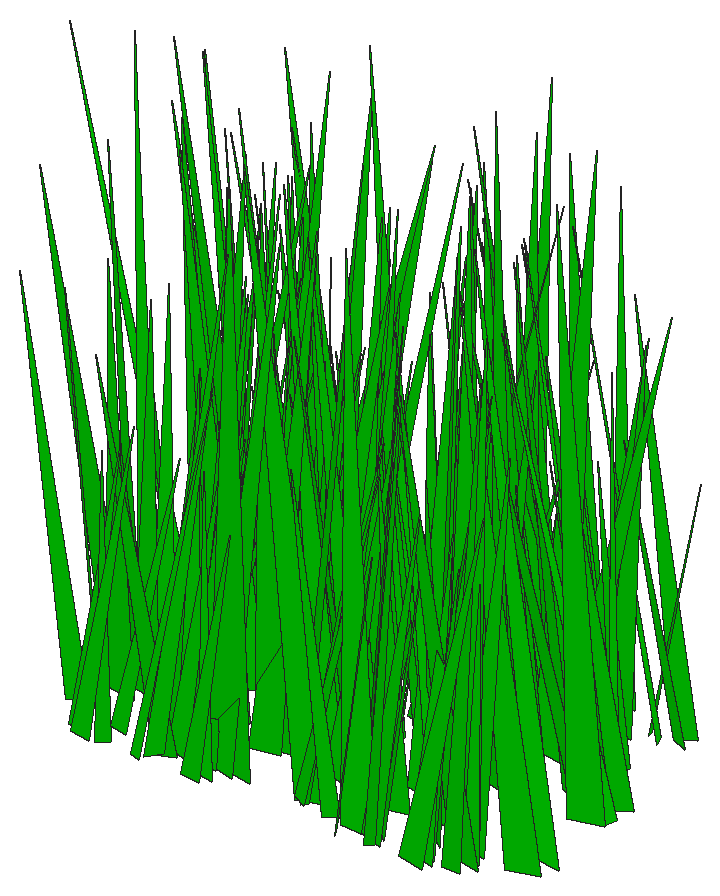
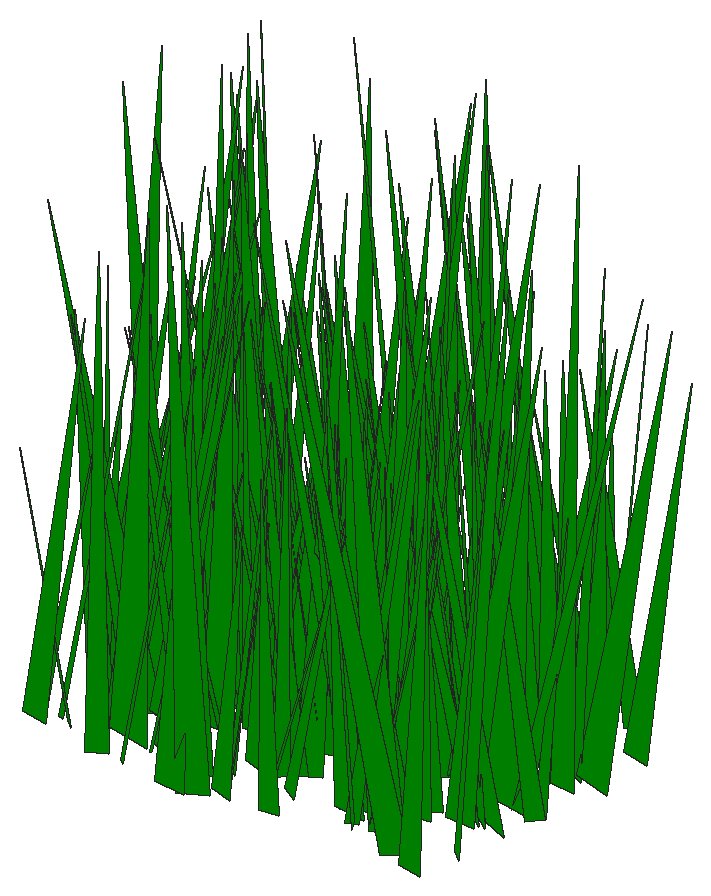
# SketchUp Ruby script. Lengths in inches.
U = 1.inch
M = Sketchup.active_model
def pt(a) = Geom::Point3d.new(a.map { |v| v * U })
def face(e, loops, mat)
  f = e.add_face(loops[0].map { |a| pt(a) })
  loops[1..].each { |l| e.add_face(l.map { |a| pt(a) }).erase! }
  f.material = f.back_material = mat if mat
  f
end
# faces: each face lists its corners as indices into pts; further lists are holes
def faces(e, pts, list, mat = nil) = list.each { |f| face(e, (f[0].is_a?(Array) ? f : [f]).map { |l| l.map { |i| pts[i] } }, mat) }
# xy, xz, yz: faces in a plane at the given z, y or x. An outline is a flat list of corners, or four numbers for a rectangle; further outlines are holes
def ring(l) = l.size == 4 ? [[l[0], l[1]], [l[2], l[1]], [l[2], l[3]], [l[0], l[3]]] : l.each_slice(2).to_a
def flat(e, list, mat, &to3) = list.each { |f| face(e, (f[0].is_a?(Array) ? f : [f]).map { |l| ring(l).map { |u, v| to3.(u, v) } }, mat) }
def xy(e, z, list, mat = nil) = flat(e, list, mat) { |x, y| [x, y, z] }
def xz(e, y, list, mat = nil) = flat(e, list, mat) { |x, z| [x, y, z] }
def yz(e, x, list, mat = nil) = flat(e, list, mat) { |y, z| [x, y, z] }
def lines(e, pts, list) = list.each { |a, b| e.add_line(pt(pts[a]), pt(pts[b])) }
# prism: a flat outline (further loops are holes) pulled along v
def prism(e, loops, v, mat = nil)
  f = face(e, loops, mat); d = Geom::Vector3d.new(v.map { |x| x * U })
  f.pushpull(f.normal.samedirection?(d) ? d.length : -d.length)
end
def box(e, o, s, mat = nil) = prism(e, [[o, [o[0] + s[0], o[1], o[2]], [o[0] + s[0], o[1] + s[1], o[2]], [o[0], o[1] + s[1], o[2]]]], [0, 0, s[2]], mat)
def at(x, y, z, deg = 0) = Geom::Transformation.translation(pt([x, y, z])) * Geom::Transformation.rotation(ORIGIN, Z_AXIS, deg.degrees)
def axes(o, x, y, z) = Geom::Transformation.new([*x, 0, *y, 0, *z, 0, *pt(o).to_a, 1])
def part(name) = M.definitions.add(name)
# library, detail: a bought-in or finely detailed component or shape, given as its bounding box
def library(name, o, s) = part(name).tap { |d| box(d.entities, o, s) }
def detail(e, o, s) = box(e.add_group.entities, o, s)
def put(e, d, t, mat = nil) = e.add_instance(d, t).tap { |i| i.material = mat if mat }
def group(e, t, mat = nil) = e.add_group.tap { |g| g.transformation = t; g.material = mat if mat }.entities
root = M.entities
M.materials.add("[Color G06]").color = [0, 204, 0]
c1 = part("fur_instance\#9")
p = [[0.8125,0,1.79],[0.67,-0.02,1.48],[0,-0.11,0],[0,0.11,0]]
faces(c1.entities,p,[[0,1,2,3]])
put(root,c1,axes([12.96,21.07,4.28],[-5.73012,0.26102,0.16531],[1.85665,0.79674,-0.75835],[0.26235,0.0625,8.97748]),"[Color G06]")
put(root,c1,axes([12.26,19.0625,4.28],[-1.91963,-0.63161,0.80341],[-4.54214,0.25727,-1.00806],[-0.41693,0.10528,7.28303]),"[Color G06]")
put(root,c1,axes([12.26,17.32,4.28],[-2.61545,0.40431,1.3874],[3.04038,0.35565,0.89688],[0.15639,-0.15259,5.76663]),"[Color G06]")
put(root,c1,axes([12.21,21.22,4.28],[-2.29903,-0.29235,0.649],[-2.03826,0.32606,0.74361],[0.65523,-0.01149,4.59037]),"[Color G06]")
put(root,c1,axes([12.65,23.98,4.28],[-4.15703,-0.11065,2.06],[-0.97542,0.60222,-0.681],[1.25616,0.10146,6.28839]),"[Color G06]")
put(root,c1,axes([12.88,18.97,4.28],[-4.33591,-0.28902,2.61767],[-2.31769,0.63388,-0.53572],[1.41126,0.15303,7.16264]),"[Color G06]")
put(root,c1,axes([12.75,19.63,4.28],[4.88864,-0.37633,3.79351],[-2.77065,-0.76039,-0.68997],[-2.45955,0.10857,8.31728]),"[Color G06]")
put(root,c1,axes([13.98,22.05,4.28],[-3.26033,0.56295,0.65909],[4.0606,0.45068,0.64862],[-0.06275,-0.08583,7.72846]),"[Color G06]")
put(root,c1,axes([13.66,22.6,4.28],[-3.93789,0.49775,2.13304],[3.7478,0.5605,0.43018],[0.85572,-0.16425,7.93188]),"[Color G06]")
put(root,c1,axes([12.92,18.2,4.28],[-1.50608,-0.5524,1.31487],[-4.01419,0.22197,0.44165],[0.59399,0.09944,6.31862]),"[Color G06]")
put(root,c1,axes([13.12,25.3,4.28],[2.44503,-0.37492,2.27674],[-2.76176,-0.38664,-0.68886],[-1.38636,0.109,5.38761]),"[Color G06]")
put(root,c1,axes([13.32,18.79,4.28],[-2.18977,-0.32853,0.08054],[-2.30074,0.30026,0.96737],[0.5101,-0.05606,4.70893]),"[Color G06]")
put(root,c1,axes([13.77,16.46,4.28],[-4.01635,-0.00671,1.65809],[-0.14527,0.57871,-0.51696],[1.10091,0.05188,5.98086]),"[Color G06]")
put(root,c1,axes([12.26,21.36,4.28],[2.70681,-0.34413,1.40695],[-2.62904,-0.36913,0.92662],[-0.25433,0.15313,5.39555]),"[Color G06]")
put(root,c1,axes([13.39,21.18,4.28],[1.14111,-0.75149,0.75161],[-5.35533,-0.16715,-1.03698],[-0.78495,0.04793,8.16748]),"[Color G06]")
put(root,c1,axes([13.24,22.27,4.28],[3.75906,0.21028,1.79588],[1.40228,-0.55012,0.84303],[-1.3234,0.01437,5.99439]),"[Color G06]")
put(root,c1,axes([13.45,18.54,4.28],[-0.80491,-0.51357,1.60388],[-3.79779,0.12824,0.45987],[0.5409,0.13618,5.61558]),"[Color G06]")
put(root,c1,axes([13.77,18.82,4.28],[-1.84737,0.50296,0.88846],[3.56898,0.26825,-0.86815],[0.79073,-0.0357,5.99413]),"[Color G06]")
put(root,c1,axes([14.68,20.36,4.28],[1.65867,-0.55788,3.72649],[-4.40961,-0.31393,-1.01465],[-1.66674,0.27537,6.3929]),"[Color G06]")
put(root,c1,axes([13.26,16.14,4.28],[1.41844,-0.3668,0.72603],[-2.67125,-0.19026,0.61586],[0.13909,0.08668,4.42381]),"[Color G06]")
put(root,c1,axes([12.75,22.33,4.28],[4.03643,0.43596,0.19433],[3.0991,-0.56107,0.80481],[-0.43207,0.04834,7.58811]),"[Color G06]")
put(root,c1,axes([13.79,22,4.28],[2.70528,0.54886,1.29202],[3.94688,-0.39018,0.58055],[-0.81336,-0.06784,7.11451]),"[Color G06]")
put(root,c1,axes([14.12,16.02,4.28],[1.85873,-0.30771,0.94847],[-2.15998,-0.27295,-0.717],[-0.77883,0.02261,4.25208]),"[Color G06]")
put(root,c1,axes([15.51,20.56,4.28],[-4.41911,-0.57542,1.84956],[-4.27521,0.61621,-0.79428],[0.53077,0.17261,9.00148]),"[Color G06]")
put(root,c1,axes([14.04,21.31,4.28],[3.29197,-0.19388,1.62443],[-1.23577,-0.48226,-1.0181],[-1.25991,-0.03358,5.24299]),"[Color G06]")
put(root,c1,axes([13.34,22.35,4.28],[3.56682,0.16153,0.78701],[1.12809,-0.50252,0.42798],[-0.58868,0.01574,5.58859]),"[Color G06]")
put(root,c1,axes([15.32,24.125,4.28],[-3.24525,-0.03887,0.44614],[-0.23336,0.45005,0.71292],[0.3352,-0.06303,4.81564]),"[Color G06]")
put(root,c1,axes([13.9,20.64,4.28],[-0.90508,0.5293,1.18172],[3.78029,0.14562,-1.02534],[0.86143,-0.08294,5.74118]),"[Color G06]")
put(root,c1,axes([13.49,15.9,4.28],[2.38084,-0.32525,0.68901],[-2.37632,-0.32851,0.5272],[-0.07825,0.08021,4.95343]),"[Color G06]")
put(root,c1,axes([15.25,20.97,4.28],[-3.56565,0.06157,1.26457],[0.60497,0.49874,1.02085],[0.73815,-0.11135,5.2719]),"[Color G06]")
put(root,c1,axes([15.17,23.18,4.28],[-0.65236,0.52819,1.4543],[3.88514,0.0718,0.89744],[-0.4473,-0.14674,5.67399]),"[Color G06]")
put(root,c1,axes([15.47,20.48,4.28],[-5.29759,0.30919,2.67583],[2.4628,0.76185,0.77892],[1.43396,-0.16621,8.54774]),"[Color G06]")
put(root,c1,axes([14.625,23.07,4.28],[-2.0021,-0.54704,1.78945],[-4.00065,0.30142,0.58655],[0.90435,0.12234,6.55637]),"[Color G06]")
put(root,c1,axes([15.48,22.54,4.28],[-4.26373,-0.01786,1.45657],[-0.05881,0.6085,0.47273],[0.9812,-0.04115,6.35778]),"[Color G06]")
put(root,c1,axes([15.9,23.62,4.28],[-2.28928,0.74824,0.34352],[5.35803,0.31578,0.74638],[-0.36983,-0.05672,8.68704]),"[Color G06]")
put(root,c1,axes([15.73,24.34,4.28],[-4.23872,-0.34946,0.84135],[-2.44431,0.59535,0.89887],[0.78903,-0.03301,7.30438]),"[Color G06]")
put(root,c1,axes([15.77,16.42,4.28],[-1.68248,-0.481,0.77083],[-3.46706,0.22199,-0.99136],[-0.37882,0.10458,5.64956]),"[Color G06]")
put(root,c1,axes([14.58,22.65,4.28],[-2.15505,0.48216,1.6815],[3.44309,0.32923,-0.98762],[1.169,-0.08082,6.00872]),"[Color G06]")
put(root,c1,axes([16.24,22.12,4.28],[-4.78365,0.22102,1.07387],[1.66265,0.667,0.77379],[0.51395,-0.10057,7.49191]),"[Color G06]")
put(root,c1,axes([13.61,22.12,4.28],[2.45655,-0.27821,0.32276],[-1.99451,-0.33323,0.91305],[0.22155,0.08491,4.64088]),"[Color G06]")
put(root,c1,axes([14.83,23.92,4.28],[-3.23172,-0.03782,2.35877],[-0.61487,0.48698,-0.98484],[1.47861,0.11985,4.74592]),"[Color G06]")
put(root,c1,axes([14.0625,16.69,4.28],[2.46534,-0.24964,0.46483],[-1.817,-0.33842,0.64792],[0.00695,0.07439,4.50727]),"[Color G06]")
put(root,c1,axes([14.98,18.02,4.28],[2.45174,0.34699,0.99179],[2.41553,-0.35415,0.89502],[-0.89305,-0.00528,5.14367]),"[Color G06]")
put(root,c1,axes([14.35,23.8,4.28],[2.33565,-0.23306,0.88241],[-1.76811,-0.31595,0.86809],[-0.12515,0.11416,4.20376]),"[Color G06]")
put(root,c1,axes([14.73,24.19,4.28],[-0.29126,0.70448,2.35628],[5.23157,0.07159,-1.01418],[0.79949,-0.21179,7.49486]),"[Color G06]")
put(root,c1,axes([14.87,19.35,4.28],[2.21677,0.63715,2.74961],[4.90744,-0.30985,-0.58979],[-0.42299,-0.25566,7.56727]),"[Color G06]")
put(root,c1,axes([14.88,17.71,4.28],[0.12518,-0.52419,0.61727],[-3.72781,-0.00741,0.96595],[0.63629,0.05972,5.53775]),"[Color G06]")
put(root,c1,axes([15.91,22.43,4.28],[1.58004,0.67476,1.87161],[4.88573,-0.24715,1.0223],[-1.05479,-0.134,7.53885]),"[Color G06]")
put(root,c1,axes([15.96,19.05,4.28],[-1.63706,0.44205,0.05051],[3.15154,0.2275,-0.55243],[0.34386,0.01949,5.30366]),"[Color G06]")
put(root,c1,axes([15.22,22.6,4.28],[2.33561,-0.30399,0.37131],[-2.12181,-0.32581,-0.82941],[-0.55866,-0.03346,4.70246]),"[Color G06]")
put(root,c1,axes([16.48,20.67,4.28],[-2.81984,-0.07576,0.83412],[-0.60957,0.39662,-0.46499],[0.48483,0.05803,4.2667]),"[Color G06]")
put(root,c1,axes([13.89,24.91,4.28],[3.68541,-0.55514,0.02064],[-3.95052,-0.50964,1.02141],[0.4922,0.06614,8.0435]),"[Color G06]")
put(root,c1,axes([15.66,24.38,4.28],[-3.21343,0.02957,2.75258],[-0.10179,0.51034,-0.89531],[1.85109,0.0794,4.72915]),"[Color G06]")
put(root,c1,axes([14.98,22.86,4.28],[3.30063,-0.17028,0.11302],[-1.18875,-0.45352,-0.94575],[-0.28938,-0.07918,5.17409]),"[Color G06]")
put(root,c1,axes([16.11,16.9,4.28],[-1.90332,0.41264,1.70378],[3.01456,0.29298,-0.62869],[0.98415,-0.09938,5.2208]),"[Color G06]")
put(root,c1,axes([16.11,23.96,4.28],[1.0184,0.61792,0.12415],[4.42297,-0.14246,0.40615],[-0.28346,-0.00278,6.78335]),"[Color G06]")
put(root,c1,axes([15.42,18.09,4.28],[1.146,-0.43319,0.1216],[-3.07365,-0.15622,0.77402],[0.45821,0.03552,4.88791]),"[Color G06]")
put(root,c1,axes([15.37,21.02,4.28],[4.42051,-0.5384,2.83898],[-4.19865,-0.62281,1.03524],[-0.94172,0.24949,8.71074]),"[Color G06]")
put(root,c1,axes([15.19,15.93,4.28],[3.87633,-0.08428,0.78886],[-0.67421,-0.53897,0.78589],[-0.43508,0.08434,5.81055]),"[Color G06]")
put(root,c1,axes([15.36,18.48,4.28],[2.4062,0.21844,0.12875],[1.55815,-0.33017,-0.69667],[0.1832,-0.06097,4.23428]),"[Color G06]")
put(root,c1,axes([16.7,19.55,4.28],[-1.96523,0.45502,0.69759],[3.21467,0.28132,-0.85023],[0.72907,-0.0139,5.62927]),"[Color G06]")
put(root,c1,axes([15.93,16.6875,4.28],[1.32443,-0.34788,1.52229],[-2.69001,-0.1614,0.99085],[0.15822,0.16803,4.10351]),"[Color G06]")
put(root,c1,axes([15.98,22.78,4.28],[2.7676,0.15744,0.35392],[1.07478,-0.38309,0.80208],[-0.41904,0.05724,4.39473]),"[Color G06]")
put(root,c1,axes([15.71,17.73,4.28],[2.09927,-0.60581,1.34054],[-4.43232,-0.28076,0.92915],[0.18236,0.15004,7.1513]),"[Color G06]")
put(root,c1,axes([16.23,23.8,4.28],[0.86128,0.37056,1.62678],[2.86235,-0.09801,-0.8204],[0.23137,-0.1669,4.0937]),"[Color G06]")
put(root,c1,axes([15.52,16.27,4.28],[4.91918,-0.33141,0.88295],[-2.3227,-0.68997,-0.8437],[-0.7761,-0.03565,8.12145]),"[Color G06]")
put(root,c1,axes([17.24,19.44,4.28],[-4.97481,0.10512,2.89123],[0.94666,0.7382,0.55535],[1.84779,-0.09519,7.49956]),"[Color G06]")
put(root,c1,axes([17,22.18,4.28],[1.85051,0.28069,1.38495],[1.98959,-0.28458,0.6875],[-0.97577,-0.04794,4.02833]),"[Color G06]")
put(root,c1,axes([16.98,17.6,4.28],[-3.95968,0.3979,3.73575],[3.36619,0.60085,0.61824],[1.74887,-0.25562,7.2683]),"[Color G06]")
put(root,c1,axes([16.875,23.3,4.28],[2.98057,0.22606,1.88785],[1.62154,-0.44932,0.46216],[-1.26266,-0.04339,5.04989]),"[Color G06]")
put(root,c1,axes([17.91,24.12,4.28],[-2.64052,-0.1973,0.83337],[-1.50876,0.35941,-0.90387],[0.19083,0.11158,4.38511]),"[Color G06]")
put(root,c1,axes([17.73,20.95,4.28],[-0.22557,-0.44507,0.26884],[-3.1239,0.02535,-1.03409],[-0.67888,0.03124,4.66906]),"[Color G06]")
put(root,c1,axes([17.66,22.26,4.28],[-2.4545,0.2512,1.33975],[1.95642,0.34401,0.59681],[0.47013,-0.12012,4.51108]),"[Color G06]")
put(root,c1,axes([17.22,16.17,4.28],[-2.20491,0.24723,1.31253],[1.74805,0.32931,-0.56615],[0.92677,-0.03295,4.19053]),"[Color G06]")
put(root,c1,axes([16.65,16.71,4.28],[1.2222,0.64069,1.0278],[4.64406,-0.1658,-0.46291],[0.12603,-0.10369,7.09066]),"[Color G06]")
put(root,c1,axes([16.49,16.94,4.28],[2.28032,0.29379,0.78568],[2.16938,-0.31285,-0.62602],[-0.09429,-0.0928,4.59765]),"[Color G06]")
put(root,c1,axes([18.48,24.125,4.28],[-2.9654,-0.01009,0.08236],[-0.06422,0.40978,0.60143],[0.0644,-0.05592,4.39234]),"[Color G06]")
put(root,c1,axes([18.08,23.12,4.28],[4.16161,-0.36074,5.30574],[-3.46542,-0.68866,0.69293],[-2.6992,0.32797,7.29074]),"[Color G06]")
put(root,c1,axes([16.33,17.875,4.28],[5.07784,-0.34171,1.57308],[-2.41626,-0.72305,-0.62051],[-1.12891,0.01058,8.40384]),"[Color G06]")
put(root,c1,axes([16.59,22.3,4.28],[1.73392,0.34497,0.83832],[2.53348,-0.23079,-0.79552],[0.12641,-0.10638,4.44446]),"[Color G06]")
put(root,c1,axes([17.2,22.59,4.28],[1.76719,0.33791,0.33893],[2.36709,-0.24772,0.80135],[-0.56592,0.01904,4.41023]),"[Color G06]")
put(root,c1,axes([16.79,23.06,4.28],[2.91983,-0.14426,1.10869],[-1.15884,-0.40834,0.71352],[-0.52691,0.09866,4.57441]),"[Color G06]")
put(root,c1,axes([16.23,22.65,4.28],[2.52262,0.67268,0.70747],[4.83457,-0.34383,-0.952],[0.34874,-0.09941,8.08017]),"[Color G06]")
put(root,c1,axes([17.58,21.16,4.28],[-0.69286,0.48236,0.25125],[3.44864,0.09829,-0.43341],[0.31757,-0.01496,5.2548]),"[Color G06]")
put(root,c1,axes([16.76,21.94,4.28],[3.1486,0.17519,0.37663],[1.20679,-0.43677,0.80263],[-0.43067,0.05689,5.00261]),"[Color G06]")
put(root,c1,axes([16.95,15.92,4.28],[1.34187,-0.3281,0.31954],[-2.35562,-0.18318,0.49048],[0.18082,0.04845,4.01839]),"[Color G06]")
put(root,c1,axes([17.7,18.3,4.28],[1.62992,-0.73322,1.23716],[-5.2655,-0.23977,-0.82852],[-0.77929,0.08655,8.18569]),"[Color G06]")
put(root,c1,axes([17.18,18.42,4.28],[3.84917,-0.10603,1.60162],[-0.61685,-0.55423,-0.90345],[-1.16019,-0.05711,5.79402]),"[Color G06]")
put(root,c1,axes([17.52,16.77,4.28],[-0.71128,-0.84139,0.99409],[-6.04525,0.10667,0.70994],[0.55219,0.08403,9.0527]),"[Color G06]")
put(root,c1,axes([17.7,25.19,4.28],[-1.03821,-0.39867,1.58422],[-2.97765,0.16618,0.44516],[0.65654,0.12325,4.52416]),"[Color G06]")
put(root,c1,axes([19.07,18.125,4.28],[-5.35733,0.3832,2.27627],[2.93912,0.75961,0.762],[1.11026,-0.16183,8.96651]),"[Color G06]")
put(root,c1,axes([17.58,19.47,4.28],[2.57756,-0.05109,1.21335],[-0.49936,-0.36991,0.58035],[-0.73753,0.07191,3.84755]),"[Color G06]")
put(root,c1,axes([18.55,20.02,4.28],[-1.51431,0.50229,1.72973],[3.78318,0.20302,0.62583],[0.04335,-0.17152,5.80631]),"[Color G06]")
put(root,c1,axes([18.31,21.91,4.28],[-1.84846,0.35056,0.63041],[2.5042,0.2633,-0.41789],[0.47618,-0.02389,4.64485]),"[Color G06]")
put(root,c1,axes([16.72,21.37,4.28],[1.87787,-0.60757,0.02188],[-4.32055,-0.25938,0.92534],[0.56283,0.03603,7.03034]),"[Color G06]")
put(root,c1,axes([16.31,23.43,4.28],[5.09908,-0.32032,0.3863],[-2.28443,-0.71162,-0.4288],[-0.35332,-0.02173,8.34756]),"[Color G06]")
put(root,c1,axes([17.1,20.97,4.28],[2.57929,-0.1867,0.39998],[-1.36356,-0.35631,0.53573],[-0.06987,0.06161,4.31018]),"[Color G06]")
put(root,c1,axes([17.1875,16.7,4.28],[2.91318,0.60824,1.81698],[4.51847,-0.40362,-0.66135],[-0.29507,-0.17565,7.81142]),"[Color G06]")
put(root,c1,axes([17.78,21.93,4.28],[3.65801,0.41797,1.66735],[2.93248,-0.53266,0.96769],[-1.27642,-0.02592,7.00156]),"[Color G06]")
put(root,c1,axes([17.56,18.11,4.28],[2.60887,0.68686,0.04497],[4.8954,-0.36207,0.89934],[-0.54576,0.03559,8.28188]),"[Color G06]")
put(root,c1,axes([18.86,19.01,4.28],[-3.9673,0.45216,2.35904],[3.46802,0.5681,0.51932],[0.98922,-0.17822,7.64033]),"[Color G06]")
put(root,c1,axes([17.25,19.79,4.28],[1.68972,-0.49268,0.92888],[-3.57629,-0.2238,0.89548],[0.2823,0.11376,5.78449]),"[Color G06]")
put(root,c1,axes([17.85,19.48,4.28],[-2.01497,-0.30445,1.75469],[-2.09803,0.32182,1.03265],[1.32037,0.04675,4.31863]),"[Color G06]")
put(root,c1,axes([17.9,21.14,4.28],[0.40404,0.67303,1.34127],[4.90526,-0.05034,-0.39894],[0.19577,-0.12767,7.2277]),"[Color G06]")
put(root,c1,axes([18.61,23.56,4.28],[-2.86793,0.30842,1.46078],[2.15269,0.42195,-0.7933],[1.10135,-0.02162,5.35447]),"[Color G06]")
put(root,c1,axes([19.21,20.47,4.28],[-3.61763,-0.0979,1.21599],[-0.60737,0.51495,0.72649],[0.88656,-0.04672,5.45958]),"[Color G06]")
put(root,c1,axes([18.27,21,4.28],[0.72144,0.59618,0.69965],[4.29534,-0.09651,-0.44665],[0.21869,-0.07119,6.46475]),"[Color G06]")
put(root,c1,axes([20.16,16.875,4.28],[-2.39087,0.78787,0.77588],[5.66085,0.32593,0.94536],[-0.38337,-0.10081,9.12043]),"[Color G06]")
put(root,c1,axes([19.41,24.58,4.28],[-2.65814,-0.04901,0.82088],[-0.262,0.37465,0.6746],[0.59713,-0.0538,3.95017]),"[Color G06]")
put(root,c1,axes([19.69,19.2,4.28],[-3.54282,0.42863,2.29234],[3.3619,0.49576,0.95742],[0.70597,-0.20984,6.94447]),"[Color G06]")
put(root,c1,axes([19.24,25.2,4.28],[0.90375,-0.37357,0.34044],[-2.60827,-0.12995,-0.91409],[-0.65248,0.00203,4.12557]),"[Color G06]")
put(root,c1,axes([18.33,23.27,4.28],[3.39408,-0.3398,1.75591],[-2.6113,-0.48018,0.60049],[-0.70653,0.14238,6.21573]),"[Color G06]")
put(root,c1,axes([19.77,24.07,4.28],[-3.49966,-0.15175,1.49867],[-1.23531,0.49727,-0.6596],[0.81469,0.10214,5.43767]),"[Color G06]")
put(root,c1,axes([19.46,19.89,4.28],[1.51345,-0.38075,1.25376],[-2.68243,-0.23494,-0.96332],[-0.98166,0.05499,4.56529]),"[Color G06]")
put(root,c1,axes([19.51,23.54,4.28],[1.14298,0.33226,1.41588],[2.43606,-0.18585,0.61718],[-0.80023,-0.09119,3.90114]),"[Color G06]")
put(root,c1,axes([19.73,20.71,4.28],[-2.40761,0.17424,1.76207],[1.50734,0.35004,0.62446],[0.82411,-0.13121,4.00569]),"[Color G06]")
put(root,c1,axes([20.625,17.94,4.28],[-3.99213,-0.17313,1.35631],[-1.39146,0.55655,-0.98771],[0.65483,0.12715,6.16986]),"[Color G06]")
put(root,c1,axes([19.86,21.9375,4.28],[0.92365,0.51379,0.73461],[3.66049,-0.13801,0.80758],[-0.6468,-0.04733,5.6195]),"[Color G06]")
put(root,c1,axes([19.13,17.65,4.28],[5.70383,0.258,2.33977],[1.80979,-0.82469,0.59129],[-1.61204,-0.01298,8.94255]),"[Color G06]")
put(root,c1,axes([21.03,21.45,4.28],[-2.19894,-0.33212,0.54175],[-2.40799,0.30085,-0.64511],[-0.07542,0.07789,4.80169]),"[Color G06]")
put(root,c1,axes([19.78,25.65,4.28],[3.2581,-0.54379,4.01468],[-4.60502,-0.46978,1.03821],[-1.10311,0.355,7.52355]),"[Color G06]")
put(root,c1,axes([20.45,25.74,4.28],[0.06349,-0.59364,0.77436],[-4.27944,-0.01348,-0.40315],[-0.27941,0.07153,6.35053]),"[Color G06]")
put(root,c1,axes([20.89,16.57,4.28],[-2.18683,0.31608,1.25533],[2.4025,0.30165,0.62376],[0.26718,-0.12537,4.66584]),"[Color G06]")
put(root,c1,axes([20.8125,20.43,4.28],[-0.26709,-0.42748,0.34561],[-3.04978,0.03276,-0.60949],[-0.38751,0.03679,4.55855]),"[Color G06]")
put(root,c1,axes([19.41,21.7,4.28],[2.32711,-0.19991,0.21211],[-1.43876,-0.32061,0.54823],[0.07292,0.05389,4.04809]),"[Color G06]")
put(root,c1,axes([21.95,24.61,4.28],[-4.92577,-0.11296,0.7384],[-0.77062,0.68877,0.62104],[0.55357,-0.04631,7.43492]),"[Color G06]")
put(root,c1,axes([19.77,20.66,4.28],[3.16918,0.09092,0.84652],[0.53893,-0.44291,0.95773],[-0.67488,0.07325,4.73999]),"[Color G06]")
put(root,c1,axes([20.375,24.75,4.28],[-2.59629,0.59084,3.00691],[4.47852,0.40757,-0.56213],[1.39411,-0.20896,7.40564]),"[Color G06]")
put(root,c1,axes([19.98,16.67,4.28],[2.38687,0.20056,0.25479],[1.39669,-0.33087,0.69193],[-0.38338,0.0433,4.10708]),"[Color G06]")
put(root,c1,axes([21.68,24.36,4.28],[-2.70456,-0.52948,0.95574],[-3.84897,0.37485,-0.47394],[0.10943,0.09836,6.95126]),"[Color G06]")
put(root,c1,axes([19.82,18.15,4.28],[1.83029,-0.44111,1.13471],[-3.24495,-0.23894,1.02153],[0.23071,0.13877,5.36577]),"[Color G06]")
put(root,c1,axes([20.73,22.18,4.28],[2.89395,0.2669,2.48485],[2.25416,-0.43191,-0.53491],[-1.16039,-0.17337,5.15799]),"[Color G06]")
put(root,c1,axes([21.49,19.87,4.28],[-2.71167,0.12095,1.26397],[1.06377,0.37607,0.9639],[0.5796,-0.12435,4.14445]),"[Color G06]")
put(root,c1,axes([19.59,20.1875,4.28],[3.8196,0.14328,0.35077],[1.04316,-0.53149,-0.43452],[-0.15037,-0.0477,5.89561]),"[Color G06]")
put(root,c1,axes([19.77,16.72,4.28],[3.23098,0.23785,0.42284],[1.7269,-0.44803,-0.5254],[-0.08443,-0.06181,5.43518]),"[Color G06]")
put(root,c1,axes([20.82,21.1,4.28],[2.58569,0.38728,1.33715],[2.7745,-0.37794,0.59022],[-0.90329,-0.05226,5.64054]),"[Color G06]")
put(root,c1,axes([20.7,20.54,4.28],[2.22503,0.2456,1.8107],[2.05179,-0.3138,-0.74234],[-0.60006,-0.16228,4.17578]),"[Color G06]")
put(root,c1,axes([22.2,25.45,4.28],[-4.24391,-0.04275,0.95294],[-0.22596,0.59429,0.81451],[0.67041,-0.07029,6.30698]),"[Color G06]")
put(root,c1,axes([21.41,22.67,4.28],[-3.67353,0.46565,3.23107],[3.73187,0.5455,0.44668],[1.37755,-0.23604,7.40626]),"[Color G06]")
put(root,c1,axes([20.78,21.36,4.28],[0.96367,-0.698,3.08578],[-5.41405,-0.12,0.65853],[0.07795,0.29419,7.58998]),"[Color G06]")
put(root,c1,axes([21.83,23.78,4.28],[-0.64936,-0.41329,0.17386],[-2.95565,0.08877,-0.41768],[-0.2484,0.02412,4.5154]),"[Color G06]")
put(root,c1,axes([21.33,22.49,4.28],[2.86578,-0.12721,1.6792],[-0.74079,-0.4275,-0.89635],[-1.24329,-0.0385,4.40462]),"[Color G06]")
put(root,c1,axes([21.92,16.39,4.28],[-2.76021,0.67236,1.59019],[4.86285,0.39964,-0.55629],[0.8563,-0.10222,8.28495]),"[Color G06]")
put(root,c1,axes([19.46,22.24,4.28],[5.84584,-0.02326,0.32425],[-0.15455,-0.81451,-0.48909],[-0.22586,-0.04478,8.7269]),"[Color G06]")
put(root,c1,axes([22.03,17.8125,4.28],[-0.34259,0.44277,1.34613],[3.29012,0.0358,0.5177],[-0.26177,-0.12952,4.74502]),"[Color G06]")
put(root,c1,axes([20.77,24.76,4.28],[4.01566,-0.19159,0.81282],[-1.29074,-0.56171,-0.96518],[-0.71934,-0.06164,6.2694]),"[Color G06]")
put(root,c1,axes([21.8,21.12,4.28],[-3.99012,-0.45838,2.95708],[-3.3888,0.6077,0.60703],[1.79888,0.12808,7.70269]),"[Color G06]")
put(root,c1,axes([23.03,22.65,4.28],[-4.6407,0.13705,0.9954],[0.91196,0.65142,-0.80572],[0.76013,0.05515,7.04376]),"[Color G06]")
put(root,c1,axes([23.125,22.95,4.28],[-4.87191,-0.50235,0.88498],[-3.55653,0.68415,0.87703],[0.82442,-0.01725,9.0133]),"[Color G06]")
put(root,c1,axes([22.75,23.11,4.28],[-1.02925,-0.54329,1.06052],[-3.92893,0.12727,-1.02784],[-0.49656,0.11913,5.93441]),"[Color G06]")
put(root,c1,axes([22.89,22.09,4.28],[-2.71587,-0.03131,0.26925],[-0.26009,0.36906,-0.92941],[0.12345,0.08862,3.96545]),"[Color G06]")
put(root,c1,axes([22.06,21.48,4.28],[0.61998,0.67684,0.69087],[4.8587,-0.09119,0.52361],[-0.40748,-0.05756,7.29453]),"[Color G06]")
put(root,c1,axes([22.4,22.71,4.28],[0.64518,0.60993,2.05217],[4.53303,-0.11375,0.70012],[-0.6845,-0.17837,6.57075]),"[Color G06]")
put(root,c1,axes([21.43,16.09,4.28],[2.89329,-0.00931,0.90833],[0.07498,-0.40141,-1.00588],[-0.60679,-0.09397,4.2068]),"[Color G06]")
put(root,c1,axes([21.53,17.07,4.28],[4.6613,0.06214,2.18268],[0.31145,-0.67914,0.73532],[-1.49477,0.05227,6.95967]),"[Color G06]")
put(root,c1,axes([20.6,23.33,4.28],[3.93519,0.14449,0.17291],[1.04259,-0.54549,-0.63926],[-0.00231,-0.06179,6.04819]),"[Color G06]")
put(root,c1,axes([23.23,22.99,4.28],[-1.43973,-0.57611,0.54015],[-4.12882,0.19409,-0.80215],[-0.39051,0.07194,6.48958]),"[Color G06]")
put(root,c1,axes([23.11,18.05,4.28],[-4.01924,0.32838,1.0158],[2.27029,0.56738,-1.00453],[0.92365,0.03431,6.88931]),"[Color G06]")
put(root,c1,axes([22.85,24.39,4.28],[0.14635,0.77284,0.89476],[5.53552,-0.03001,0.95504],[-0.6582,-0.08053,8.231]),"[Color G06]")
put(root,c1,axes([22.53,21.38,4.28],[-4.08045,-0.53502,4.11368],[-4.42725,0.60988,-0.6975],[1.64202,0.31483,8.34197]),"[Color G06]")
put(root,c1,axes([23.51,23.73,4.28],[-4.57486,0.09208,1.3798],[0.75746,0.64582,0.65902],[0.84533,-0.08037,6.87681]),"[Color G06]")
put(root,c1,axes([22.91,20.32,4.28],[-2.29353,-0.44048,0.54314],[-3.13446,0.32371,0.59189],[0.53426,0.00821,5.80419]),"[Color G06]")
put(root,c1,axes([23.02,21.86,4.28],[1.6403,0.45864,2.91702],[3.61635,-0.28237,0.55767],[-1.24462,-0.216,5.46474]),"[Color G06]")
put(root,c1,axes([22.1,18.83,4.28],[-1.88756,0.6868,2.98285],[5.12876,0.31277,-1.0232],[1.39168,-0.22115,7.81648]),"[Color G06]")
put(root,c1,axes([22.57,19.91,4.28],[2.36049,-0.17005,1.22501],[-1.14871,-0.34844,-0.6119],[-0.91616,-0.00125,3.92347]),"[Color G06]")
put(root,c1,axes([21.97,21.54,4.28],[2.45162,-0.40867,1.53104],[-3.09063,-0.33851,0.67498],[-0.29404,0.15063,5.67063]),"[Color G06]")
put(root,c1,axes([22.92,18.2,4.28],[-1.45813,-0.40699,1.05785],[-2.94946,0.21473,0.40925],[0.56587,0.07052,4.85901]),"[Color G06]")
put(root,c1,axes([22.97,25.49,4.28],[3.56362,-0.34479,3.67102],[-3.03116,-0.54839,0.65595],[-1.72016,0.25204,6.44931]),"[Color G06]")
put(root,c1,axes([22.5,16.08,4.28],[3.81162,0.28702,1.70804],[1.978,-0.55488,0.85134],[-1.27676,-0.00278,6.41807]),"[Color G06]")
put(root,c1,axes([23.58,24.33,4.28],[-2.63782,0.08887,0.58059],[0.5401,0.3646,-0.92981],[0.51514,0.0728,3.94783]),"[Color G06]")
put(root,c1,axes([22.36,16.29,4.28],[1.90781,0.37687,1.16169],[2.81205,-0.25707,-0.73557],[-0.03024,-0.12822,4.88931]),"[Color G06]")
put(root,c1,axes([22.54,19.03,4.28],[2.27967,0.48996,0.31208],[3.50021,-0.31922,0.45851],[-0.37103,-0.00105,6.24301]),"[Color G06]")
put(root,c1,axes([22.47,16.625,4.28],[2.8452,0.07515,0.97221],[0.6638,-0.39601,-0.82279],[-0.52246,-0.09388,4.24904]),"[Color G06]")
put(root,c1,axes([23,19.08,4.28],[3.7766,-0.62246,2.39021],[-4.51762,-0.55895,-0.77688],[-1.44027,0.12104,8.70429]),"[Color G06]")
put(root,c1,axes([24.8125,24.625,4.28],[-4.81291,-0.00111,1.07624],[0.05982,0.67561,0.67734],[0.71766,-0.06373,7.1613]),"[Color G06]")
put(root,c1,axes([22.37,18.24,4.28],[4.4631,-0.05871,0.92848],[-0.33685,-0.62356,-0.91263],[-0.67062,-0.07752,6.6376]),"[Color G06]")
put(root,c1,axes([25.51,20.67,4.28],[-4.32795,-0.38594,0.12299],[-2.76602,0.60165,-0.54246],[-0.12641,0.04881,7.65879]),"[Color G06]")
put(root,c1,axes([23.94,20.83,4.28],[-2.69896,0.05257,1.48644],[0.52317,0.39495,0.51744],[0.92604,-0.06993,4.03995]),"[Color G06]")
put(root,c1,axes([24.04,20.12,4.28],[2.26604,0.26458,2.21827],[1.94843,-0.36839,0.60148],[-1.41649,-0.08348,4.37603]),"[Color G06]")
put(root,c1,axes([23.9375,22.91,4.28],[-2.82923,-0.14419,1.48674],[-0.97382,0.4182,0.51971],[1.05377,-0.00066,4.47195]),"[Color G06]")
put(root,c1,axes([23,23.96,4.28],[3.30379,0.37643,0.23876],[2.64809,-0.45748,1.00524],[-0.54802,0.05876,6.29673]),"[Color G06]")
put(root,c1,axes([23.31,22.29,4.28],[0.67739,0.82341,1.9976],[6.04511,-0.08167,-0.71178],[0.33312,-0.19233,8.85464]),"[Color G06]")
put(root,c1,axes([24.73,22.3125,4.28],[-2.79248,-0.15437,0.6098],[-1.06724,0.39283,0.50686],[0.503,-0.02353,4.46086]),"[Color G06]")
put(root,c1,axes([24.83,21.1,4.28],[-4.35122,-0.36164,1.46454],[-2.54509,0.6219,0.74998],[1.09927,0.00839,7.53345]),"[Color G06]")
put(root,c1,axes([24.93,16.78,4.28],[-2.71976,-0.5868,0.06777],[-4.20028,0.37897,0.41995],[0.26057,-0.01597,7.4768]),"[Color G06]")
put(root,c1,axes([23.72,17.22,4.28],[-4.89225,-0.21928,3.87033],[-1.53738,0.77068,0.67501],[2.61059,0.04293,7.65053]),"[Color G06]")
put(root,c1,axes([23.71,24.34,4.28],[0.56166,-0.55325,0.98743],[-4.00492,-0.06833,0.69051],[0.37164,0.09976,5.9489]),"[Color G06]")
put(root,c1,axes([23.92,16.31,4.28],[-0.47917,0.47811,0.18085],[3.37248,0.06877,-0.9253],[0.63,-0.00449,5.09081]),"[Color G06]")
put(root,c1,axes([23.99,16.5,4.28],[2.05711,0.2642,1.27441],[2.04107,-0.28825,-0.49476],[-0.38833,-0.11548,4.15045]),"[Color G06]")
put(root,c1,axes([25.32,25.0625,4.28],[-2.82134,0.40298,1.6225],[3.06539,0.38996,0.78062],[0.36501,-0.16009,5.98548]),"[Color G06]")
put(root,c1,axes([25.32,24.8,4.28],[-2.47136,-0.25085,0.09336],[-1.77957,0.34273,0.5591],[0.27032,-0.0371,4.53418]),"[Color G06]")
put(root,c1,axes([24.96,22.9375,4.28],[1.49105,-0.33448,1.4298],[-2.37283,-0.23824,-0.87507],[-1.01908,0.06533,4.12949]),"[Color G06]")
put(root,c1,axes([25.57,21.6,4.28],[1.9502,0.37579,3.7841],[3.17379,-0.37493,0.62349],[-1.89735,-0.24091,4.93246]),"[Color G06]")
put(root,c1,axes([26.47,20.63,4.28],[-4.44474,0.18802,0.42474],[1.37387,0.615,0.84006],[0.10648,-0.08656,6.89093]),"[Color G06]")
put(root,c1,axes([24.94,21.13,4.28],[-2.6495,-0.22662,2.38555],[-2.034,0.38907,-0.80035],[1.02548,0.18619,4.57598]),"[Color G06]")
put(root,c1,axes([23.2,23.1,4.28],[3.69384,-0.46654,0.18192],[-3.33832,-0.51136,0.76353],[0.25332,0.06415,7.40941]),"[Color G06]")
put(root,c1,axes([25.71,21.72,4.28],[-1.82285,-0.30803,1.09014],[-2.32432,0.2465,-0.68041],[0.096,0.11915,4.22602]),"[Color G06]")
put(root,c1,axes([24.72,17.05,4.28],[-2.75125,0.50402,3.45454],[3.96117,0.44549,-0.41963],[1.64796,-0.22937,6.77599]),"[Color G06]")
put(root,c1,axes([23.85,16,4.28],[2.49689,-0.41464,0.52922],[-2.98409,-0.33918,0.92192],[0.24954,0.09288,5.72943]),"[Color G06]")
put(root,c1,axes([24.99,16.97,4.28],[-1.41556,0.29409,1.3881],[2.17197,0.22106,-0.43244],[0.77003,-0.08289,3.77152]),"[Color G06]")
put(root,c1,axes([24.44,24.77,4.28],[2.61814,0.10346,0.40459],[0.68633,-0.36272,0.73441],[-0.3908,0.05613,4.00023]),"[Color G06]")
put(root,c1,axes([26.5,18.04,4.28],[-4.83986,0.47441,0.68511],[3.34985,0.67683,-0.97871],[0.75042,0.0384,8.78752]),"[Color G06]")
put(root,c1,axes([26.35,17.34,4.28],[-2.2882,0.68431,0.75544],[4.92787,0.3134,0.72979],[-0.23174,-0.09252,8.05955]),"[Color G06]")
put(root,c1,axes([24.87,16.33,4.28],[3.60888,0.40915,1.93655],[2.97677,-0.52853,0.43626],[-1.19454,-0.08097,6.93778]),"[Color G06]")
put(root,c1,axes([25.27,22.28,4.28],[3.5617,-0.14685,2.27489],[-0.9347,-0.53999,-0.73534],[-1.59753,-0.01145,5.5021]),"[Color G06]")
put(root,c1,axes([24.66,17.38,4.28],[1.82547,-0.46421,1.87802],[-3.55631,-0.24447,0.78001],[-0.11642,0.18904,5.62046]),"[Color G06]")
put(root,c1,axes([26.32,21.29,4.28],[-1.49354,0.43742,0.64344],[3.14319,0.19684,0.92571],[-0.3814,-0.09075,5.10935]),"[Color G06]")
put(root,c1,axes([25.98,20.27,4.28],[-2.7441,0.64683,3.53494],[5.15051,0.39186,0.69409],[0.76328,-0.31881,8.02499]),"[Color G06]")
